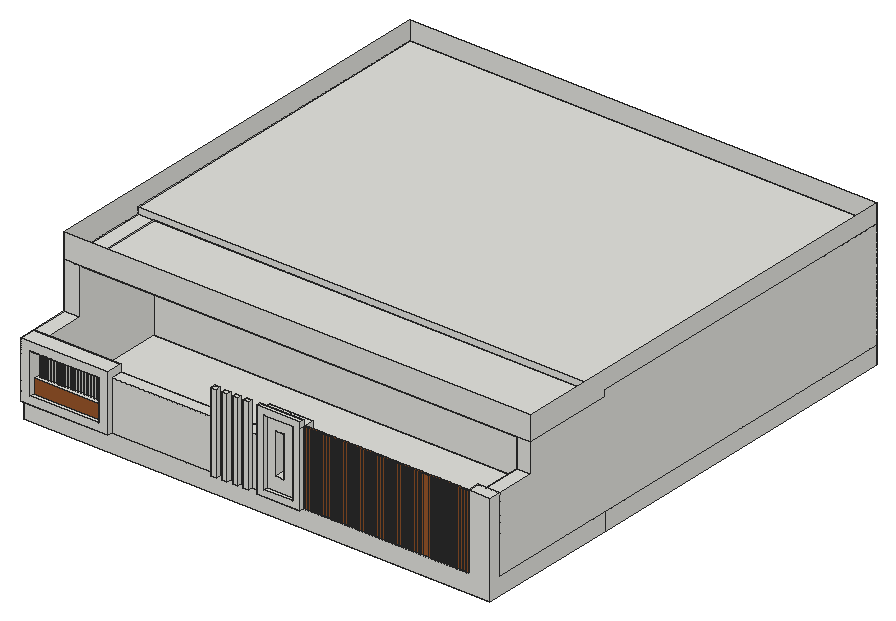
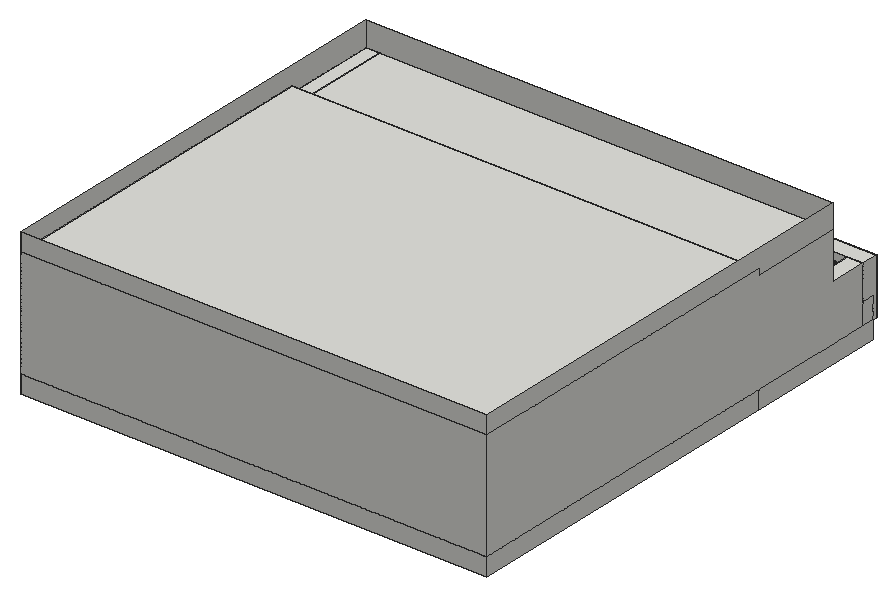
# SketchUp Ruby script. Lengths in inches.
U = 1.inch
M = Sketchup.active_model
def pt(a) = Geom::Point3d.new(a.map { |v| v * U })
def face(e, loops, mat)
  f = e.add_face(loops[0].map { |a| pt(a) })
  loops[1..].each { |l| e.add_face(l.map { |a| pt(a) }).erase! }
  f.material = f.back_material = mat if mat
  f
end
# faces: each face lists its corners as indices into pts; further lists are holes
def faces(e, pts, list, mat = nil) = list.each { |f| face(e, (f[0].is_a?(Array) ? f : [f]).map { |l| l.map { |i| pts[i] } }, mat) }
# xy, xz, yz: faces in a plane at the given z, y or x. An outline is a flat list of corners, or four numbers for a rectangle; further outlines are holes
def ring(l) = l.size == 4 ? [[l[0], l[1]], [l[2], l[1]], [l[2], l[3]], [l[0], l[3]]] : l.each_slice(2).to_a
def flat(e, list, mat, &to3) = list.each { |f| face(e, (f[0].is_a?(Array) ? f : [f]).map { |l| ring(l).map { |u, v| to3.(u, v) } }, mat) }
def xy(e, z, list, mat = nil) = flat(e, list, mat) { |x, y| [x, y, z] }
def xz(e, y, list, mat = nil) = flat(e, list, mat) { |x, z| [x, y, z] }
def yz(e, x, list, mat = nil) = flat(e, list, mat) { |y, z| [x, y, z] }
def lines(e, pts, list) = list.each { |a, b| e.add_line(pt(pts[a]), pt(pts[b])) }
# prism: a flat outline (further loops are holes) pulled along v
def prism(e, loops, v, mat = nil)
  f = face(e, loops, mat); d = Geom::Vector3d.new(v.map { |x| x * U })
  f.pushpull(f.normal.samedirection?(d) ? d.length : -d.length)
end
def box(e, o, s, mat = nil) = prism(e, [[o, [o[0] + s[0], o[1], o[2]], [o[0] + s[0], o[1] + s[1], o[2]], [o[0], o[1] + s[1], o[2]]]], [0, 0, s[2]], mat)
def at(x, y, z, deg = 0) = Geom::Transformation.translation(pt([x, y, z])) * Geom::Transformation.rotation(ORIGIN, Z_AXIS, deg.degrees)
def axes(o, x, y, z) = Geom::Transformation.new([*x, 0, *y, 0, *z, 0, *pt(o).to_a, 1])
def part(name) = M.definitions.add(name)
# library, detail: a bought-in or finely detailed component or shape, given as its bounding box
def library(name, o, s) = part(name).tap { |d| box(d.entities, o, s) }
def detail(e, o, s) = box(e.add_group.entities, o, s)
def put(e, d, t, mat = nil) = e.add_instance(d, t).tap { |i| i.material = mat if mat }
def group(e, t, mat = nil) = e.add_group.tap { |g| g.transformation = t; g.material = mat if mat }.entities
root = M.entities
M.materials.add("[Wood Cherry Original]").color = [152, 86, 42]
xy(root,-40.1875,[[0,6.4375,676.6875,213.8125],[0,213.8125,676.6875,706.875]])
xy(root,-13.9375,[[0,0,14.3125,6.4375],[14.3125,0,127.06,6.4375],[276.6875,0,284.5,6.4375],[292.1875,0,300,6.4375],[307.6875,0,315.5,6.4375],
  [323.1875,0,331,6.4375],[342.5,0,405.6875,6.4375],[0,6.4375,405.6875,23.875],[405.6875,6.4375,645.125,23.875],[0,23.875,23.1875,213.8125],
  [23.1875,23.875,656.9375,213.8125],[656.9375,23.875,676.6875,213.8125],[0,213.8125,676.6875,706.875]])
xy(root,-5.3125,[[353.1875,0,394.9375,6.4375]])
xy(root,-2.4375,[[14.3125,0,113.68,6.4375]])
xy(root,13.85,[[365.27,6.4375,377.75,23.875]])
xy(root,17.6875,[[[14.3125,6.4375,113.68,23.875],[16.82,13.45,18.82,16.82],[20.95,13.45,22.95,16.82],[25.07,13.45,27.07,16.82],[29.2,13.45,31.2,16.82],[33.32,13.45,35.32,16.82],[37.45,13.45,39.45,16.82],[41.57,13.45,43.57,16.82],[45.7,13.45,47.7,16.82],[49.82,13.45,51.82,16.82],[53.95,13.45,55.95,16.82],[58.07,13.45,60.07,16.82],[62.76,13.45,64.76,16.82],[67.45,13.45,69.45,16.82],[72.13,13.45,74.13,16.82],[76.82,13.45,78.82,16.82],[81.51,13.45,83.51,16.82],[86.2,13.45,88.2,16.82],[90.88,13.45,92.88,16.82],[95.57,13.45,97.57,16.82],[100.26,13.45,102.26,16.82],[104.95,13.45,106.95,16.82],[109.63,13.45,111.63,16.82]],[114.32,13.45,116.32,16.82],[119.01,13.45,121.01,16.82],[123.7,13.45,125.7,16.82],[128.38,13.45,130.38,16.82],
  [133.07,13.45,135.07,16.82],[137.76,13.45,139.76,16.82],[142.45,13.45,144.45,16.82],[147.13,13.45,149.13,16.82],[151.82,13.45,153.82,16.82]])
xy(root,56.6875,[[14.3125,0,113.68,23.875]])
xy(root,57.9375,[[16.82,13.45,18.82,16.82],[20.95,13.45,22.95,16.82],[25.07,13.45,27.07,16.82],[29.2,13.45,31.2,16.82],[33.32,13.45,35.32,16.82],
  [37.45,13.45,39.45,16.82],[41.57,13.45,43.57,16.82],[45.7,13.45,47.7,16.82],[49.82,13.45,51.82,16.82],[53.95,13.45,55.95,16.82],
  [58.07,13.45,60.07,16.82],[62.76,13.45,64.76,16.82],[67.45,13.45,69.45,16.82],[72.13,13.45,74.13,16.82],[76.82,13.45,78.82,16.82],
  [81.51,13.45,83.51,16.82],[86.2,13.45,88.2,16.82],[90.88,13.45,92.88,16.82],[95.57,13.45,97.57,16.82],[100.26,13.45,102.26,16.82],
  [104.95,13.45,106.95,16.82],[109.63,13.45,111.63,16.82]])
xy(root,58.375,[[127.06,6.4375,342.5,23.875]])
xy(root,67.8125,[[0,0,127.06,23.875],[0,23.875,23.1875,79.8125]])
xy(root,73.1875,[[365.27,6.4375,377.75,23.875]])
xy(root,92.25,[[353.1875,0,394.9375,6.4375],[342.5,6.4375,365.27,23.875],[365.27,6.4375,376.0625,23.875],[376.0625,6.4375,405.6875,23.875]])
xy(root,93.75,[[645.125,6.4375,676.6875,23.875],[656.9375,23.875,676.6875,79.8125]])
xy(root,100.75,[[276.6875,0,284.5,6.4375],[292.1875,0,300,6.4375],[307.6875,0,315.5,6.4375],[323.1875,0,331,6.4375],[342.5,0,405.6875,6.4375]])
xy(root,135.0625,[[0,79.8125,23.1875,213.8125],[23.1875,79.8125,656.9375,213.8125],[656.9375,79.8125,676.6875,213.8125]])
xy(root,144,[[0,213.8125,676.6875,706.875]])
xz(root,0,[[[0,-13.9375,127.06,67.8125],[14.3125,-2.4375,113.68,56.6875]],[276.6875,-13.9375,284.5,100.75],[292.1875,-13.9375,300,100.75],[307.6875,-13.9375,315.5,100.75],[323.1875,-13.9375,331,100.75],
  [[342.5,-13.9375,405.6875,100.75],[353.1875,-5.3125,394.9375,92.25]]])
xz(root,6.4375,[[0,-40.1875,676.6875,-40.1875,676.6875,93.75,645.125,93.75,645.125,-13.9375,0,-13.9375],[127.06,-13.9375,276.6875,58.375],[276.6875,-13.9375,284.5,58.375],[284.5,-13.9375,292.1875,58.375],[292.1875,-13.9375,300,58.375],
  [300,-13.9375,307.6875,58.375],[307.6875,-13.9375,315.5,58.375],[315.5,-13.9375,323.1875,58.375],[323.1875,-13.9375,331,58.375],[331,-13.9375,342.5,58.375],
  [342.5,-13.9375,342.5,92.25,353.1875,92.25,353.1875,-5.3125,394.9375,-5.3125,394.9375,92.25,405.6875,92.25,405.6875,-13.9375],[[353.1875,-5.3125,394.9375,92.25],[365.27,13.85,377.75,73.1875]],[276.6875,58.375,284.5,100.75],[292.1875,58.375,300,100.75],[307.6875,58.375,315.5,100.75],
  [323.1875,58.375,331,100.75],[342.5,92.25,405.6875,100.75]])
xz(root,6.4375,[[14.3125,-2.4375,113.68,17.6875]],"[Wood Cherry Original]")
xz(root,13.45,[[16.82,17.6875,18.82,57.9375],[20.95,17.6875,22.95,57.9375],[25.07,17.6875,27.07,57.9375],[29.2,17.6875,31.2,57.9375],[33.32,17.6875,35.32,57.9375],
  [37.45,17.6875,39.45,57.9375],[41.57,17.6875,43.57,57.9375],[45.7,17.6875,47.7,57.9375],[49.82,17.6875,51.82,57.9375],[53.95,17.6875,55.95,57.9375],
  [58.07,17.6875,60.07,57.9375],[62.76,17.6875,64.76,57.9375],[67.45,17.6875,69.45,57.9375],[72.13,17.6875,74.13,57.9375],[76.82,17.6875,78.82,57.9375],
  [81.51,17.6875,83.51,57.9375],[86.2,17.6875,88.2,57.9375],[90.88,17.6875,92.88,57.9375],[95.57,17.6875,97.57,57.9375],[100.26,17.6875,102.26,57.9375],
  [104.95,17.6875,106.95,57.9375],[109.63,17.6875,111.63,57.9375]])
xz(root,16.82,[[16.82,17.6875,18.82,57.9375],[20.95,17.6875,22.95,57.9375],[25.07,17.6875,27.07,57.9375],[29.2,17.6875,31.2,57.9375],[33.32,17.6875,35.32,57.9375],
  [37.45,17.6875,39.45,57.9375],[41.57,17.6875,43.57,57.9375],[45.7,17.6875,47.7,57.9375],[49.82,17.6875,51.82,57.9375],[53.95,17.6875,55.95,57.9375],
  [58.07,17.6875,60.07,57.9375],[62.76,17.6875,64.76,57.9375],[67.45,17.6875,69.45,57.9375],[72.13,17.6875,74.13,57.9375],[76.82,17.6875,78.82,57.9375],
  [81.51,17.6875,83.51,57.9375],[86.2,17.6875,88.2,57.9375],[90.88,17.6875,92.88,57.9375],[95.57,17.6875,97.57,57.9375],[100.26,17.6875,102.26,57.9375],
  [104.95,17.6875,106.95,57.9375],[109.63,17.6875,111.63,57.9375]])
xz(root,23.875,[[0,-13.9375,23.1875,-13.9375,23.1875,17.6875,14.3125,17.6875,14.3125,17.9375,0,17.9375],[23.1875,-13.9375,23.1875,17.6875,113.68,17.6875,113.68,17.9375,127.06,17.9375,127.06,58.375,342.5,58.375,342.5,92.25,365.27,92.25,365.27,13.85,377.75,13.85,377.75,73.1875,376.0625,73.1875,376.0625,92.25,405.6875,92.25,405.6875,-13.9375],[645.125,-13.9375,656.9375,93.75],[656.9375,-13.9375,676.6875,93.75],[14.3125,17.6875,23.1875,56.6875],
  [0,17.9375,0,67.8125,23.1875,67.8125,23.1875,56.6875,14.3125,56.6875,14.3125,17.9375],[113.68,17.9375,113.68,56.6875,23.1875,56.6875,23.1875,67.8125,127.06,67.8125,127.06,17.9375],[365.27,73.1875,376.0625,92.25]])
xz(root,79.8125,[[0,67.8125,23.1875,135.0625],[656.9375,93.75,676.6875,135.0625],[0,135.0625,676.6875,170.875]])
xz(root,213.8125,[[0,-40.1875,676.6875,-13.9375],[23.1875,-13.9375,656.9375,135.0625],[0,135.0625,676.6875,144]])
xz(root,706.875,[[0,-40.1875,676.6875,-13.9375],[0,-13.9375,676.6875,144],[0,144,676.6875,170.875]])
yz(root,0,[[6.4375,-40.1875,213.8125,-13.9375],[213.8125,-40.1875,706.875,-13.9375],[0,-13.9375,0,67.8125,23.875,67.8125,23.875,17.9375,6.4375,17.9375,6.4375,-13.9375],[6.4375,-13.9375,23.875,17.9375],[23.875,-13.9375,23.875,67.8125,79.8125,67.8125,79.8125,135.0625,213.8125,135.0625,213.8125,144,706.875,144,706.875,-13.9375],
  [79.8125,135.0625,79.8125,170.875,706.875,170.875,706.875,144,213.8125,144,213.8125,135.0625]])
yz(root,14.3125,[[0,-2.4375,6.4375,-2.4375,6.4375,17.6875,23.875,17.6875,23.875,56.6875,0,56.6875]])
yz(root,16.82,[[13.45,17.6875,16.82,57.9375]])
yz(root,18.82,[[13.45,17.6875,16.82,57.9375]])
yz(root,20.95,[[13.45,17.6875,16.82,57.9375]])
yz(root,22.95,[[13.45,17.6875,16.82,57.9375]])
yz(root,23.1875,[[23.875,-13.9375,213.8125,-13.9375,213.8125,135.0625,79.8125,135.0625,79.8125,67.8125,23.875,67.8125]])
yz(root,25.07,[[13.45,17.6875,16.82,57.9375]])
yz(root,27.07,[[13.45,17.6875,16.82,57.9375]])
yz(root,29.2,[[13.45,17.6875,16.82,57.9375]])
yz(root,31.2,[[13.45,17.6875,16.82,57.9375]])
yz(root,33.32,[[13.45,17.6875,16.82,57.9375]])
yz(root,35.32,[[13.45,17.6875,16.82,57.9375]])
yz(root,37.45,[[13.45,17.6875,16.82,57.9375]])
yz(root,39.45,[[13.45,17.6875,16.82,57.9375]])
yz(root,41.57,[[13.45,17.6875,16.82,57.9375]])
yz(root,43.57,[[13.45,17.6875,16.82,57.9375]])
yz(root,45.7,[[13.45,17.6875,16.82,57.9375]])
yz(root,47.7,[[13.45,17.6875,16.82,57.9375]])
yz(root,49.82,[[13.45,17.6875,16.82,57.9375]])
yz(root,51.82,[[13.45,17.6875,16.82,57.9375]])
yz(root,53.95,[[13.45,17.6875,16.82,57.9375]])
yz(root,55.95,[[13.45,17.6875,16.82,57.9375]])
yz(root,58.07,[[13.45,17.6875,16.82,57.9375]])
yz(root,60.07,[[13.45,17.6875,16.82,57.9375]])
yz(root,62.76,[[13.45,17.6875,16.82,57.9375]])
yz(root,64.76,[[13.45,17.6875,16.82,57.9375]])
yz(root,67.45,[[13.45,17.6875,16.82,57.9375]])
yz(root,69.45,[[13.45,17.6875,16.82,57.9375]])
yz(root,72.13,[[13.45,17.6875,16.82,57.9375]])
yz(root,74.13,[[13.45,17.6875,16.82,57.9375]])
yz(root,76.82,[[13.45,17.6875,16.82,57.9375]])
yz(root,78.82,[[13.45,17.6875,16.82,57.9375]])
yz(root,81.51,[[13.45,17.6875,16.82,57.9375]])
yz(root,83.51,[[13.45,17.6875,16.82,57.9375]])
yz(root,86.2,[[13.45,17.6875,16.82,57.9375]])
yz(root,88.2,[[13.45,17.6875,16.82,57.9375]])
yz(root,90.88,[[13.45,17.6875,16.82,57.9375]])
yz(root,92.88,[[13.45,17.6875,16.82,57.9375]])
yz(root,95.57,[[13.45,17.6875,16.82,57.9375]])
yz(root,97.57,[[13.45,17.6875,16.82,57.9375]])
yz(root,100.26,[[13.45,17.6875,16.82,57.9375]])
yz(root,102.26,[[13.45,17.6875,16.82,57.9375]])
yz(root,104.95,[[13.45,17.6875,16.82,57.9375]])
yz(root,106.95,[[13.45,17.6875,16.82,57.9375]])
yz(root,109.63,[[13.45,17.6875,16.82,57.9375]])
yz(root,111.63,[[13.45,17.6875,16.82,57.9375]])
yz(root,113.68,[[0,-2.4375,0,56.6875,23.875,56.6875,23.875,17.6875,6.4375,17.6875,6.4375,-2.4375]])
yz(root,127.06,[[0,-13.9375,6.4375,-13.9375,6.4375,58.375,23.875,58.375,23.875,67.8125,0,67.8125],[6.4375,17.9375,23.875,58.375]])
yz(root,276.6875,[[0,-13.9375,6.4375,100.75]])
yz(root,284.5,[[0,-13.9375,6.4375,100.75]])
yz(root,292.1875,[[0,-13.9375,6.4375,100.75]])
yz(root,300,[[0,-13.9375,6.4375,100.75]])
yz(root,307.6875,[[0,-13.9375,6.4375,100.75]])
yz(root,315.5,[[0,-13.9375,6.4375,100.75]])
yz(root,323.1875,[[0,-13.9375,6.4375,100.75]])
yz(root,331,[[0,-13.9375,6.4375,100.75]])
yz(root,342.5,[[0,-13.9375,6.4375,100.75],[6.4375,58.375,23.875,92.25]])
yz(root,353.1875,[[0,-5.3125,6.4375,92.25]])
yz(root,365.27,[[6.4375,13.85,23.875,73.1875]])
yz(root,377.75,[[6.4375,13.85,23.875,73.1875]])
yz(root,394.9375,[[0,-5.3125,6.4375,92.25]])
yz(root,405.6875,[[0,-13.9375,6.4375,92.25],[6.4375,-13.9375,23.875,92.25],[0,92.25,6.4375,100.75]])
yz(root,645.125,[[6.4375,-13.9375,23.875,93.75]])
yz(root,656.9375,[[23.875,-13.9375,23.875,93.75,79.8125,93.75,79.8125,135.0625,213.8125,135.0625,213.8125,-13.9375]])
yz(root,676.6875,[[6.4375,-40.1875,213.8125,-40.1875,213.8125,-13.9375,23.875,-13.9375,23.875,93.75,6.4375,93.75],[213.8125,-40.1875,706.875,-13.9375],[23.875,-13.9375,706.875,-13.9375,706.875,144,213.8125,144,213.8125,135.0625,79.8125,135.0625,79.8125,93.75,23.875,93.75],[79.8125,135.0625,213.8125,135.0625,213.8125,144,706.875,144,706.875,170.875,79.8125,170.875]])
p = [[14.3125,6.4375,-13.9375],[14.3125,6.4375,-2.4375],[113.68,6.4375,17.9375],[127.06,6.4375,17.9375],[0,6.4375,17.9375],[14.3125,6.4375,17.9375]]
lines(root,p,[[0,1],[2,3],[4,5]])
g1 = group(root,at(406.25,6.4375,-13.9375),"[Wood Cherry Original]")
xy(g1,0,[[0,0,3.5,3],[5.5,0,7.625,3],[9.625,0,11.75,3],[13.75,0,15.875,3],[17.875,0,20,3],
  [22,0,24.125,3],[26.125,0,28.25,3],[30.25,0,32.375,3],[34.375,0,36.5,3],[38.5,0,40.625,3],
  [42.625,0,44.75,3],[46.75,0,48.875,3],[50.875,0,53,3],[55,0,57.125,3],[59.125,0,61.25,3],
  [63.25,0,65.375,3],[67.375,0,69.5,3],[71.5,0,73.625,3],[75.625,0,77.75,3],[79.75,0,81.875,3],
  [83.875,0,86,3],[88,0,90.125,3],[92.125,0,94.25,3],[96.25,0,98.375,3],[100.375,0,102.5,3],
  [104.5,0,106.625,3],[108.625,0,110.75,3],[112.75,0,114.875,3],[116.875,0,119,3],[121,0,123.125,3],
  [125.125,0,127.25,3],[129.25,0,131.375,3],[133.375,0,135.5,3],[137.5,0,139.625,3],[141.625,0,143.75,3],
  [145.75,0,147.875,3],[149.875,0,152,3],[154,0,156.125,3],[158.125,0,160.25,3],[162.25,0,164.375,3],
  [166.375,0,168.5,3],[170.5,0,181.625,3],[183.625,0,185.875,3],[187.875,0,190.125,3],[192.125,0,194.375,3],
  [196.375,0,198.625,3],[200.625,0,202.875,3],[204.875,0,207.125,3],[209.125,0,211.375,3],[213.375,0,215.625,3],
  [217.625,0,219.875,3],[221.875,0,224.125,3],[226.125,0,228.375,3],[230.375,0,232.625,3],[234.625,0,236.875,3],
  [238.875,0,239.4375,3]])
xy(g1,106.1875,[[0,0,3.5,3],[5.5,0,7.625,3],[9.625,0,11.75,3],[13.75,0,15.875,3],[17.875,0,20,3],
  [22,0,24.125,3],[26.125,0,28.25,3],[30.25,0,32.375,3],[34.375,0,36.5,3],[38.5,0,40.625,3],
  [42.625,0,44.75,3],[46.75,0,48.875,3],[50.875,0,53,3],[55,0,57.125,3],[59.125,0,61.25,3],
  [63.25,0,65.375,3],[67.375,0,69.5,3],[71.5,0,73.625,3],[75.625,0,77.75,3],[79.75,0,81.875,3],
  [83.875,0,86,3],[88,0,90.125,3],[92.125,0,94.25,3],[96.25,0,98.375,3],[100.375,0,102.5,3],
  [104.5,0,106.625,3],[108.625,0,110.75,3],[112.75,0,114.875,3],[116.875,0,119,3],[121,0,123.125,3],
  [125.125,0,127.25,3],[129.25,0,131.375,3],[133.375,0,135.5,3],[137.5,0,139.625,3],[141.625,0,143.75,3],
  [145.75,0,147.875,3],[149.875,0,152,3],[154,0,156.125,3],[158.125,0,160.25,3],[162.25,0,164.375,3],
  [166.375,0,168.5,3],[170.5,0,181.625,3],[183.625,0,185.875,3],[187.875,0,190.125,3],[192.125,0,194.375,3],
  [196.375,0,198.625,3],[200.625,0,202.875,3],[204.875,0,207.125,3],[209.125,0,211.375,3],[213.375,0,215.625,3],
  [217.625,0,219.875,3],[221.875,0,224.125,3],[226.125,0,228.375,3],[230.375,0,232.625,3],[234.625,0,236.875,3],
  [238.875,0,239.4375,3]])
xz(g1,0,[[0,0,3.5,106.1875],[5.5,0,7.625,106.1875],[9.625,0,11.75,106.1875],[13.75,0,15.875,106.1875],[17.875,0,20,106.1875],
  [22,0,24.125,106.1875],[26.125,0,28.25,106.1875],[30.25,0,32.375,106.1875],[34.375,0,36.5,106.1875],[38.5,0,40.625,106.1875],
  [42.625,0,44.75,106.1875],[46.75,0,48.875,106.1875],[50.875,0,53,106.1875],[55,0,57.125,106.1875],[59.125,0,61.25,106.1875],
  [63.25,0,65.375,106.1875],[67.375,0,69.5,106.1875],[71.5,0,73.625,106.1875],[75.625,0,77.75,106.1875],[79.75,0,81.875,106.1875],
  [83.875,0,86,106.1875],[88,0,90.125,106.1875],[92.125,0,94.25,106.1875],[96.25,0,98.375,106.1875],[100.375,0,102.5,106.1875],
  [104.5,0,106.625,106.1875],[108.625,0,110.75,106.1875],[112.75,0,114.875,106.1875],[116.875,0,119,106.1875],[121,0,123.125,106.1875],
  [125.125,0,127.25,106.1875],[129.25,0,131.375,106.1875],[133.375,0,135.5,106.1875],[137.5,0,139.625,106.1875],[141.625,0,143.75,106.1875],
  [145.75,0,147.875,106.1875],[149.875,0,152,106.1875],[154,0,156.125,106.1875],[158.125,0,160.25,106.1875],[162.25,0,164.375,106.1875],
  [166.375,0,168.5,106.1875],[170.5,0,172.25,106.1875],[172.25,0,181.625,106.1875],[183.625,0,185.875,106.1875],[187.875,0,190.125,106.1875],
  [192.125,0,194.375,106.1875],[196.375,0,198.625,106.1875],[200.625,0,202.875,106.1875],[204.875,0,207.125,106.1875],[209.125,0,211.375,106.1875],
  [213.375,0,215.625,106.1875],[217.625,0,219.875,106.1875],[221.875,0,224.125,106.1875],[226.125,0,228.375,106.1875],[230.375,0,232.625,106.1875],
  [234.625,0,236.875,106.1875],[238.875,0,239.4375,106.1875]])
xz(g1,3,[[0,0,3.5,106.1875],[3.5,0,5.5,106.1875],[5.5,0,7.625,106.1875],[7.625,0,9.625,106.1875],[9.625,0,11.75,106.1875],
  [11.75,0,13.75,106.1875],[13.75,0,15.875,106.1875],[15.875,0,17.875,106.1875],[17.875,0,20,106.1875],[20,0,22,106.1875],
  [22,0,24.125,106.1875],[24.125,0,26.125,106.1875],[26.125,0,28.25,106.1875],[28.25,0,30.25,106.1875],[30.25,0,32.375,106.1875],
  [32.375,0,34.375,106.1875],[34.375,0,36.5,106.1875],[36.5,0,38.5,106.1875],[38.5,0,40.625,106.1875],[40.625,0,42.625,106.1875],
  [42.625,0,44.75,106.1875],[44.75,0,46.75,106.1875],[46.75,0,48.875,106.1875],[48.875,0,50.875,106.1875],[50.875,0,53,106.1875],
  [53,0,55,106.1875],[55,0,57.125,106.1875],[57.125,0,59.125,106.1875],[59.125,0,61.25,106.1875],[61.25,0,63.25,106.1875],
  [63.25,0,65.375,106.1875],[65.375,0,67.375,106.1875],[67.375,0,69.5,106.1875],[69.5,0,71.5,106.1875],[71.5,0,73.625,106.1875],
  [73.625,0,75.625,106.1875],[75.625,0,77.75,106.1875],[77.75,0,79.75,106.1875],[79.75,0,81.875,106.1875],[81.875,0,83.875,106.1875],
  [83.875,0,86,106.1875],[86,0,88,106.1875],[88,0,90.125,106.1875],[90.125,0,92.125,106.1875],[92.125,0,94.25,106.1875],
  [94.25,0,96.25,106.1875],[96.25,0,98.375,106.1875],[98.375,0,100.375,106.1875],[100.375,0,102.5,106.1875],[102.5,0,104.5,106.1875],
  [104.5,0,106.625,106.1875],[106.625,0,108.625,106.1875],[108.625,0,110.75,106.1875],[110.75,0,112.75,106.1875],[112.75,0,114.875,106.1875],
  [114.875,0,116.875,106.1875],[116.875,0,119,106.1875],[119,0,121,106.1875],[121,0,123.125,106.1875],[123.125,0,125.125,106.1875],
  [125.125,0,127.25,106.1875],[127.25,0,129.25,106.1875],[129.25,0,131.375,106.1875],[131.375,0,133.375,106.1875],[133.375,0,135.5,106.1875],
  [135.5,0,137.5,106.1875],[137.5,0,139.625,106.1875],[139.625,0,141.625,106.1875],[141.625,0,143.75,106.1875],[143.75,0,145.75,106.1875],
  [145.75,0,147.875,106.1875],[147.875,0,149.875,106.1875],[149.875,0,152,106.1875],[152,0,154,106.1875],[154,0,156.125,106.1875],
  [156.125,0,158.125,106.1875],[158.125,0,160.25,106.1875],[160.25,0,162.25,106.1875],[162.25,0,164.375,106.1875],[164.375,0,166.375,106.1875],
  [166.375,0,168.5,106.1875],[168.5,0,170.5,106.1875],[170.5,0,181.625,106.1875],[181.625,0,183.625,106.1875],[183.625,0,185.875,106.1875],
  [185.875,0,187.875,106.1875],[187.875,0,190.125,106.1875],[190.125,0,192.125,106.1875],[192.125,0,194.375,106.1875],[194.375,0,196.375,106.1875],
  [196.375,0,198.625,106.1875],[198.625,0,200.625,106.1875],[200.625,0,202.875,106.1875],[202.875,0,204.875,106.1875],[204.875,0,207.125,106.1875],
  [207.125,0,209.125,106.1875],[209.125,0,211.375,106.1875],[211.375,0,213.375,106.1875],[213.375,0,215.625,106.1875],[215.625,0,217.625,106.1875],
  [217.625,0,219.875,106.1875],[219.875,0,221.875,106.1875],[221.875,0,224.125,106.1875],[224.125,0,226.125,106.1875],[226.125,0,228.375,106.1875],
  [228.375,0,230.375,106.1875],[230.375,0,232.625,106.1875],[232.625,0,234.625,106.1875],[234.625,0,236.875,106.1875],[236.875,0,238.875,106.1875],
  [238.875,0,239.4375,106.1875]])
yz(g1,0,[[0,0,3,106.1875]])
yz(g1,3.5,[[0,0,3,106.1875]])
yz(g1,5.5,[[0,0,3,106.1875]])
yz(g1,7.625,[[0,0,3,106.1875]])
yz(g1,9.625,[[0,0,3,106.1875]])
yz(g1,11.75,[[0,0,3,106.1875]])
yz(g1,13.75,[[0,0,3,106.1875]])
yz(g1,15.875,[[0,0,3,106.1875]])
yz(g1,17.875,[[0,0,3,106.1875]])
yz(g1,20,[[0,0,3,106.1875]])
yz(g1,22,[[0,0,3,106.1875]])
yz(g1,24.125,[[0,0,3,106.1875]])
yz(g1,26.125,[[0,0,3,106.1875]])
yz(g1,28.25,[[0,0,3,106.1875]])
yz(g1,30.25,[[0,0,3,106.1875]])
yz(g1,32.375,[[0,0,3,106.1875]])
yz(g1,34.375,[[0,0,3,106.1875]])
yz(g1,36.5,[[0,0,3,106.1875]])
yz(g1,38.5,[[0,0,3,106.1875]])
yz(g1,40.625,[[0,0,3,106.1875]])
yz(g1,42.625,[[0,0,3,106.1875]])
yz(g1,44.75,[[0,0,3,106.1875]])
yz(g1,46.75,[[0,0,3,106.1875]])
yz(g1,48.875,[[0,0,3,106.1875]])
yz(g1,50.875,[[0,0,3,106.1875]])
yz(g1,53,[[0,0,3,106.1875]])
yz(g1,55,[[0,0,3,106.1875]])
yz(g1,57.125,[[0,0,3,106.1875]])
yz(g1,59.125,[[0,0,3,106.1875]])
yz(g1,61.25,[[0,0,3,106.1875]])
yz(g1,63.25,[[0,0,3,106.1875]])
yz(g1,65.375,[[0,0,3,106.1875]])
yz(g1,67.375,[[0,0,3,106.1875]])
yz(g1,69.5,[[0,0,3,106.1875]])
yz(g1,71.5,[[0,0,3,106.1875]])
yz(g1,73.625,[[0,0,3,106.1875]])
yz(g1,75.625,[[0,0,3,106.1875]])
yz(g1,77.75,[[0,0,3,106.1875]])
yz(g1,79.75,[[0,0,3,106.1875]])
yz(g1,81.875,[[0,0,3,106.1875]])
yz(g1,83.875,[[0,0,3,106.1875]])
yz(g1,86,[[0,0,3,106.1875]])
yz(g1,88,[[0,0,3,106.1875]])
yz(g1,90.125,[[0,0,3,106.1875]])
yz(g1,92.125,[[0,0,3,106.1875]])
yz(g1,94.25,[[0,0,3,106.1875]])
yz(g1,96.25,[[0,0,3,106.1875]])
yz(g1,98.375,[[0,0,3,106.1875]])
yz(g1,100.375,[[0,0,3,106.1875]])
yz(g1,102.5,[[0,0,3,106.1875]])
yz(g1,104.5,[[0,0,3,106.1875]])
yz(g1,106.625,[[0,0,3,106.1875]])
yz(g1,108.625,[[0,0,3,106.1875]])
yz(g1,110.75,[[0,0,3,106.1875]])
yz(g1,112.75,[[0,0,3,106.1875]])
yz(g1,114.875,[[0,0,3,106.1875]])
yz(g1,116.875,[[0,0,3,106.1875]])
yz(g1,119,[[0,0,3,106.1875]])
yz(g1,121,[[0,0,3,106.1875]])
yz(g1,123.125,[[0,0,3,106.1875]])
yz(g1,125.125,[[0,0,3,106.1875]])
yz(g1,127.25,[[0,0,3,106.1875]])
yz(g1,129.25,[[0,0,3,106.1875]])
yz(g1,131.375,[[0,0,3,106.1875]])
yz(g1,133.375,[[0,0,3,106.1875]])
yz(g1,135.5,[[0,0,3,106.1875]])
yz(g1,137.5,[[0,0,3,106.1875]])
yz(g1,139.625,[[0,0,3,106.1875]])
yz(g1,141.625,[[0,0,3,106.1875]])
yz(g1,143.75,[[0,0,3,106.1875]])
yz(g1,145.75,[[0,0,3,106.1875]])
yz(g1,147.875,[[0,0,3,106.1875]])
yz(g1,149.875,[[0,0,3,106.1875]])
yz(g1,152,[[0,0,3,106.1875]])
yz(g1,154,[[0,0,3,106.1875]])
yz(g1,156.125,[[0,0,3,106.1875]])
yz(g1,158.125,[[0,0,3,106.1875]])
yz(g1,160.25,[[0,0,3,106.1875]])
yz(g1,162.25,[[0,0,3,106.1875]])
yz(g1,164.375,[[0,0,3,106.1875]])
yz(g1,166.375,[[0,0,3,106.1875]])
yz(g1,168.5,[[0,0,3,106.1875]])
yz(g1,170.5,[[0,0,3,106.1875]])
yz(g1,181.625,[[0,0,3,106.1875]])
yz(g1,183.625,[[0,0,3,106.1875]])
yz(g1,185.875,[[0,0,3,106.1875]])
yz(g1,187.875,[[0,0,3,106.1875]])
yz(g1,190.125,[[0,0,3,106.1875]])
yz(g1,192.125,[[0,0,3,106.1875]])
yz(g1,194.375,[[0,0,3,106.1875]])
yz(g1,196.375,[[0,0,3,106.1875]])
yz(g1,198.625,[[0,0,3,106.1875]])
yz(g1,200.625,[[0,0,3,106.1875]])
yz(g1,202.875,[[0,0,3,106.1875]])
yz(g1,204.875,[[0,0,3,106.1875]])
yz(g1,207.125,[[0,0,3,106.1875]])
yz(g1,209.125,[[0,0,3,106.1875]])
yz(g1,211.375,[[0,0,3,106.1875]])
yz(g1,213.375,[[0,0,3,106.1875]])
yz(g1,215.625,[[0,0,3,106.1875]])
yz(g1,217.625,[[0,0,3,106.1875]])
yz(g1,219.875,[[0,0,3,106.1875]])
yz(g1,221.875,[[0,0,3,106.1875]])
yz(g1,224.125,[[0,0,3,106.1875]])
yz(g1,226.125,[[0,0,3,106.1875]])
yz(g1,228.375,[[0,0,3,106.1875]])
yz(g1,230.375,[[0,0,3,106.1875]])
yz(g1,232.625,[[0,0,3,106.1875]])
yz(g1,234.625,[[0,0,3,106.1875]])
yz(g1,236.875,[[0,0,3,106.1875]])
yz(g1,238.875,[[0,0,3,106.1875]])
yz(g1,239.4375,[[0,0,3,106.1875]])
